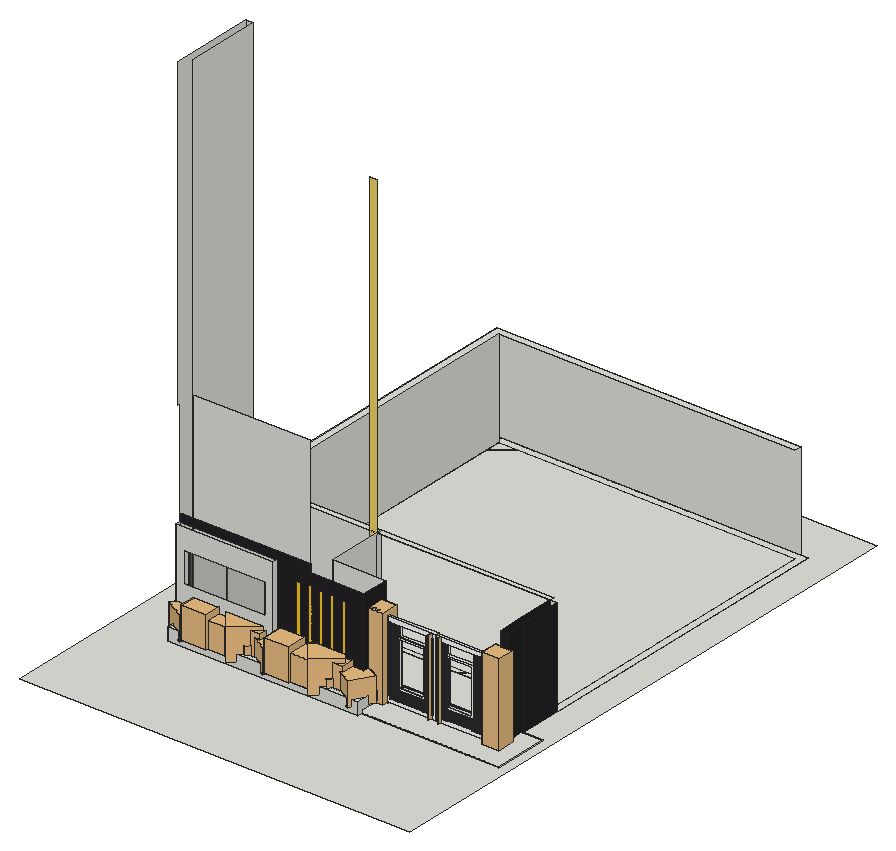
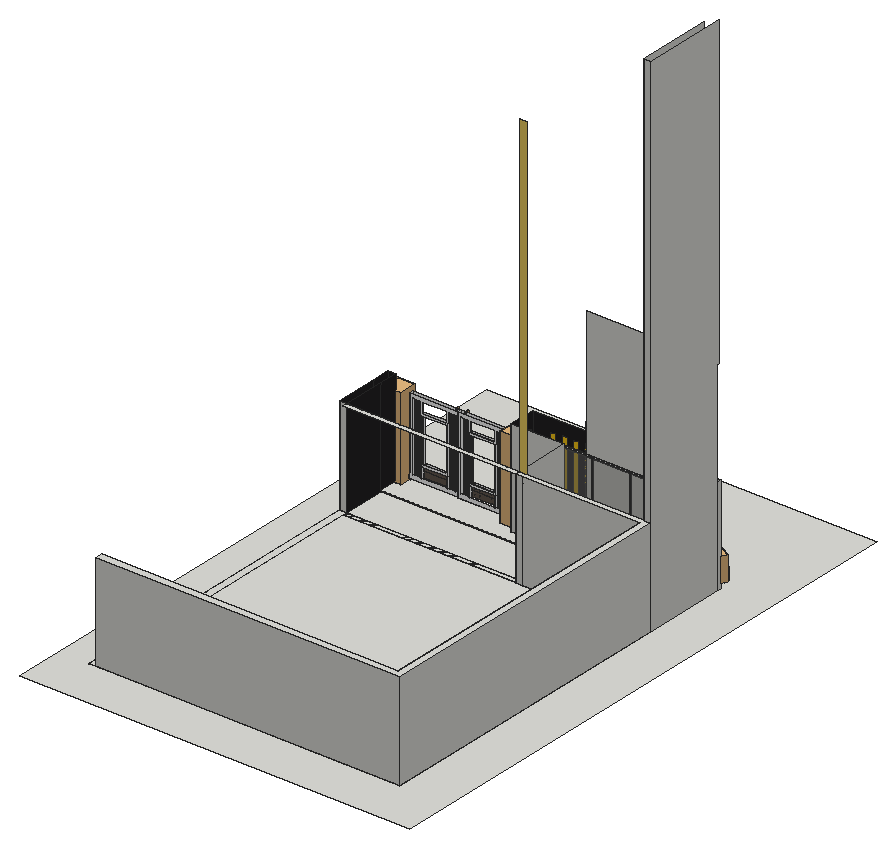
# SketchUp Ruby script. Lengths in inches.
U = 1.inch
M = Sketchup.active_model
def pt(a) = Geom::Point3d.new(a.map { |v| v * U })
def face(e, loops, mat)
  f = e.add_face(loops[0].map { |a| pt(a) })
  loops[1..].each { |l| e.add_face(l.map { |a| pt(a) }).erase! }
  f.material = f.back_material = mat if mat
  f
end
# faces: each face lists its corners as indices into pts; further lists are holes
def faces(e, pts, list, mat = nil) = list.each { |f| face(e, (f[0].is_a?(Array) ? f : [f]).map { |l| l.map { |i| pts[i] } }, mat) }
# xy, xz, yz: faces in a plane at the given z, y or x. An outline is a flat list of corners, or four numbers for a rectangle; further outlines are holes
def ring(l) = l.size == 4 ? [[l[0], l[1]], [l[2], l[1]], [l[2], l[3]], [l[0], l[3]]] : l.each_slice(2).to_a
def flat(e, list, mat, &to3) = list.each { |f| face(e, (f[0].is_a?(Array) ? f : [f]).map { |l| ring(l).map { |u, v| to3.(u, v) } }, mat) }
def xy(e, z, list, mat = nil) = flat(e, list, mat) { |x, y| [x, y, z] }
def xz(e, y, list, mat = nil) = flat(e, list, mat) { |x, z| [x, y, z] }
def yz(e, x, list, mat = nil) = flat(e, list, mat) { |y, z| [x, y, z] }
def lines(e, pts, list) = list.each { |a, b| e.add_line(pt(pts[a]), pt(pts[b])) }
# prism: a flat outline (further loops are holes) pulled along v
def prism(e, loops, v, mat = nil)
  f = face(e, loops, mat); d = Geom::Vector3d.new(v.map { |x| x * U })
  f.pushpull(f.normal.samedirection?(d) ? d.length : -d.length)
end
def box(e, o, s, mat = nil) = prism(e, [[o, [o[0] + s[0], o[1], o[2]], [o[0] + s[0], o[1] + s[1], o[2]], [o[0], o[1] + s[1], o[2]]]], [0, 0, s[2]], mat)
def at(x, y, z, deg = 0) = Geom::Transformation.translation(pt([x, y, z])) * Geom::Transformation.rotation(ORIGIN, Z_AXIS, deg.degrees)
def axes(o, x, y, z) = Geom::Transformation.new([*x, 0, *y, 0, *z, 0, *pt(o).to_a, 1])
def part(name) = M.definitions.add(name)
# library, detail: a bought-in or finely detailed component or shape, given as its bounding box
def library(name, o, s) = part(name).tap { |d| box(d.entities, o, s) }
def detail(e, o, s) = box(e.add_group.entities, o, s)
def put(e, d, t, mat = nil) = e.add_instance(d, t).tap { |i| i.material = mat if mat }
def group(e, t, mat = nil) = e.add_group.tap { |g| g.transformation = t; g.material = mat if mat }.entities
root = M.entities
M.materials.add("Glass_Mirror_3").color = [244, 212, 100]
M.materials.add("Marble_07_1K").color = [36, 34, 36]
M.materials.add("Material__1").color = [95, 70, 46]
M.materials.add("Metal_Perforated_08_1K").color = [255, 206, 27]
M.materials.add("[Color M00]").color = [255, 255, 255]
M.materials.add("[Color_000]").color = [255, 255, 255]
M.materials.add("[Color_C20]").color = [102, 91, 81]
M.materials.add("[Translucent Glass Gray]").color = [128, 128, 128]
M.materials["[Translucent Glass Gray]"].alpha = 0.29
c1 = library("Areca palm plant",[0,0,0],[49.1,36.6,54.46])
c2 = part("W1")
xy(c2.entities,15,[[0,0,2,198]])
xy(c2.entities,102.0625,[[0,0,2,198]],"[Color M00]")
xz(c2.entities,0,[[0,15,2,102.0625]],"[Color M00]")
xz(c2.entities,198,[[0,15,2,102.0625]])
yz(c2.entities,0,[[0.84,16,39.43,101.0625],[40.28,16,78.87,101.0625],[79.71,16,118.3,101.0625],[119.14,16,157.73,101.0625],[158.58,16,197.16,101.0625]])
yz(c2.entities,0,[[[0,15,198,102.0625],[0.84,16,197.16,101.0625]],[39.43,16,40.28,101.0625],[78.87,16,79.71,101.0625],[118.3,16,119.14,101.0625],[157.73,16,158.58,101.0625]],"[Color M00]")
yz(c2.entities,2,[[0.84,16,39.43,101.0625],[40.28,16,78.87,101.0625],[79.71,16,118.3,101.0625],[119.14,16,157.73,101.0625],[158.58,16,197.16,101.0625]])
yz(c2.entities,2,[[[0,15,198,102.0625],[0.84,16,197.16,101.0625]],[39.43,16,40.28,101.0625],[78.87,16,79.71,101.0625],[118.3,16,119.14,101.0625],[157.73,16,158.58,101.0625]],"[Color M00]")
c3 = library("Group\#74",[-84.69,-90.07,-0.36],[176.51,175.13,171.4])
c4 = library("Group20\#1",[-20.81,-17.08,3.79],[39.86,39.43,37.51])
c5 = library("Group\#130",[-7.34,-1.2,0],[38.67,35.81,49.04])
c6 = library("Group38\#2",[14.01,28.44,-23.43],[18.58,18.32,38.89])
c7 = part("PLANTS (1)")
put(c7.entities,c1,axes([38.49,169.84,6.02],[0.45017,-0.56191,0],[0.66137,0.52986,0],[0,0,0.72]))
put(c7.entities,c1,axes([38.49,68.02,6.02],[0.45017,-0.56191,0],[0.66137,0.52986,0],[0,0,0.72]))
put(c7.entities,c2,axes([76.68,11.43,-0.0625],[1,0,0],[0,1.18586,0],[0,0,1]),"[Translucent Glass Gray]")
put(c7.entities,c3,axes([59.61,184.54,5.99],[-0.04961,-0.08593,0],[0.08593,-0.04961,0],[0,0,0.10522]))
put(c7.entities,c3,axes([59.61,204.61,5.99],[-0.04961,-0.08593,0],[0.08593,-0.04961,0],[0,0,0.10522]))
put(c7.entities,c3,axes([59.61,157.29,5.99],[-0.04961,-0.08593,0],[0.08593,-0.04961,0],[0,0,0.10522]))
put(c7.entities,c4,axes([63.65,91.4,4.71],[0,0.85,0],[-0.85,0,0],[0,0,0.85]))
put(c7.entities,c5,axes([69.62,101.34,7.93],[0,0.79,0],[-0.79,0,0],[0,0,0.79]))
put(c7.entities,c6,axes([40.58,10.27,28.11],[0.8848,0,0],[0,0.94674,0],[0,0,0.85826]))
put(c7.entities,c3,axes([59.61,55.48,5.99],[-0.04961,-0.08593,0],[0.08593,-0.04961,0],[0,0,0.10522]))
put(c7.entities,c3,axes([59.61,82.73,5.99],[-0.04961,-0.08593,0],[0.08593,-0.04961,0],[0,0,0.10522]))
put(c7.entities,c3,axes([61.875,132.66,6.01],[-0.08133,-0.14087,0],[0.14087,-0.08133,0],[0,0,0.1725]))
put(c7.entities,c3,axes([59.61,102.79,5.99],[-0.04961,-0.08593,0],[0.08593,-0.04961,0],[0,0,0.10522]))
put(c7.entities,c3,axes([61.875,27.22,6.01],[-0.08133,-0.14087,0],[0.14087,-0.08133,0],[0,0,0.1725]))
put(c7.entities,c3,axes([61.875,234.47,6.01],[-0.08133,-0.14087,0],[0.14087,-0.08133,0],[0,0,0.1725]))
put(c7.entities,c5,axes([69.62,203.15,7.93],[0,0.79,0],[-0.79,0,0],[0,0,0.79]))
put(c7.entities,c4,axes([63.65,193.21,4.71],[0,0.85,0],[-0.85,0,0],[0,0,0.85]))
put(c7.entities,c6,axes([40.58,112.08,28.11],[0.8848,0,0],[0,0.94674,0],[0,0,0.85826]))
g1 = group(c7.entities,at(44.68,11.43,-0.0625))
xy(g1,0,[[0,0,6,234.8],[30,0,36,234.8]])
xy(g1,3,[[6,0,30,234.8]])
xy(g1,7,[[6,5,30,229.8]],"Material__1")
xy(g1,15,[[[0,0,36,234.8],[6,5,30,229.8]]])
xz(g1,0,[[0,0,6,0,6,3,30,3,30,0,36,0,36,15,0,15]])
xz(g1,5,[[6,7,30,15]])
xz(g1,229.8,[[6,7,30,15]])
xz(g1,234.8,[[0,0,0,15,36,15,36,0,30,0,30,3,6,3,6,0]])
yz(g1,0,[[0,0,234.8,15]])
yz(g1,6,[[0,0,234.8,3],[5,7,229.8,15]])
yz(g1,30,[[0,0,234.8,3],[5,7,229.8,15]])
yz(g1,36,[[0,0,234.8,15]])
c8 = library("Gate pillar",[0,0,0],[97.06,71.13,326.45])
c9 = library("Gate pull handle",[-0.01,0,0],[1.26,2.875,48])
c10 = part("Gate slat")
xy(c10.entities,0,[[0.39,114.16,6.3,114.17]])
xy(c10.entities,0,[[0.39,0,6.3,114.16]],"[Color_C20]")
xy(c10.entities,0.39,[[0.39,0,0.79,114.17],[0.98,0,2.07,114.17],[2.36,0,3.2,114.17],[3.59,0,4.37,114.17],[4.56,0,5.71,114.17],
  [5.91,0,6.3,114.17]],"[Color_C20]")
xy(c10.entities,0.79,[[0.39,0,0.79,114.17],[0.98,0,2.07,114.17],[2.36,0,3.2,114.17],[3.59,0,4.37,114.17],[4.56,0,5.71,114.17],
  [5.91,0,6.3,114.17]],"[Color_C20]")
xy(c10.entities,0.99,[[1.13,0,1.21,114.16],[1.87,0,1.94,114.16],[2.61,0,2.68,114.16],[3.35,0,3.42,114.16],[4.08,0,4.16,114.16],
  [4.82,0,4.9,114.16],[5.5625,0,5.63,114.16],[6.3,0,6.37,114.16]],"[Color_C20]")
xy(c10.entities,1.18,[[0.39,114.16,3.35,114.17],[3.35,114.16,6.3,114.17]])
xy(c10.entities,1.18,[[0.39,0,1.13,114.16],[1.21,0,1.87,114.16],[1.94,0,2.61,114.16],[2.68,0,3.35,114.16],[3.42,0,4.08,114.16],
  [4.16,0,4.82,114.16],[4.9,0,5.5625,114.16],[5.63,0,6.3,114.16]],"[Color_C20]")
xz(c10.entities,0,[[[0.39,0,6.3,0,6.3,0.39,5.91,0.39,5.91,0.79,6.3,0.79,6.3,1.18,5.63,1.18,5.63,0.99,5.5625,0.99,5.5625,1.18,4.9,1.18,4.9,0.99,4.82,0.99,4.82,1.18,4.16,1.18,4.16,0.99,4.08,0.99,4.08,1.18,3.42,1.18,3.42,0.99,3.35,0.99,3.35,1.18,2.68,1.18,2.68,0.99,2.61,0.99,2.61,1.18,1.94,1.18,1.94,0.99,1.87,0.99,1.87,1.18,1.21,1.18,1.21,0.99,1.13,0.99,1.13,1.18,0.39,1.18,0.39,0.79,0.79,0.79,0.79,0.39,0.39,0.39],[4.56,0.39,5.71,0.79],[0.98,0.39,2.07,0.79],[2.36,0.39,3.2,0.79],[3.59,0.39,4.37,0.79]],[6.3,0.99,6.37,1.18]],"[Color_C20]")
xz(c10.entities,114.16,[[1.13,0.99,1.21,1.18],[1.87,0.99,1.94,1.18],[2.61,0.99,2.68,1.18],[3.35,0.99,3.42,1.18],[4.08,0.99,4.16,1.18],
  [4.82,0.99,4.9,1.18],[5.5625,0.99,5.63,1.18]],"[Color_C20]")
xz(c10.entities,114.17,[[[0.39,0,0.39,0.39,0.79,0.39,0.79,0.79,0.39,0.79,0.39,1.18,6.3,1.18,6.3,0.79,5.91,0.79,5.91,0.39,6.3,0.39,6.3,0],[4.56,0.39,5.71,0.79],[0.98,0.39,2.07,0.79],[2.36,0.39,3.2,0.79],[3.59,0.39,4.37,0.79]]],"[Color_C20]")
yz(c10.entities,0.39,[[114.16,0,114.17,0.39],[114.16,0.79,114.17,1.18]])
yz(c10.entities,0.39,[[0,0,114.16,0.39],[0,0.79,114.16,1.18]],"[Color_C20]")
yz(c10.entities,0.79,[[0,0.39,114.17,0.79]],"[Color_C20]")
yz(c10.entities,0.98,[[0,0.39,114.17,0.79]],"[Color_C20]")
yz(c10.entities,1.13,[[0,0.99,114.16,1.18]],"[Color_C20]")
yz(c10.entities,1.21,[[0,0.99,114.16,1.18]],"[Color_C20]")
yz(c10.entities,1.87,[[0,0.99,114.16,1.18]],"[Color_C20]")
yz(c10.entities,1.94,[[0,0.99,114.16,1.18]],"[Color_C20]")
yz(c10.entities,2.07,[[0,0.39,114.17,0.79]],"[Color_C20]")
yz(c10.entities,2.36,[[0,0.39,114.17,0.79]],"[Color_C20]")
yz(c10.entities,2.61,[[0,0.99,114.16,1.18]],"[Color_C20]")
yz(c10.entities,2.68,[[0,0.99,114.16,1.18]],"[Color_C20]")
yz(c10.entities,3.2,[[0,0.39,114.17,0.79]],"[Color_C20]")
yz(c10.entities,3.35,[[0,0.99,114.16,1.18]],"[Color_C20]")
yz(c10.entities,3.42,[[0,0.99,114.16,1.18]],"[Color_C20]")
yz(c10.entities,3.59,[[0,0.39,114.17,0.79]],"[Color_C20]")
yz(c10.entities,4.08,[[0,0.99,114.16,1.18]],"[Color_C20]")
yz(c10.entities,4.16,[[0,0.99,114.16,1.18]],"[Color_C20]")
yz(c10.entities,4.37,[[0,0.39,114.17,0.79]],"[Color_C20]")
yz(c10.entities,4.56,[[0,0.39,114.17,0.79]],"[Color_C20]")
yz(c10.entities,4.82,[[0,0.99,114.16,1.18]],"[Color_C20]")
yz(c10.entities,4.9,[[0,0.99,114.16,1.18]],"[Color_C20]")
yz(c10.entities,5.5625,[[0,0.99,114.16,1.18]],"[Color_C20]")
yz(c10.entities,5.63,[[0,0.99,114.16,1.18]],"[Color_C20]")
yz(c10.entities,5.71,[[0,0.39,114.17,0.79]],"[Color_C20]")
yz(c10.entities,5.91,[[0,0.39,114.17,0.79]],"[Color_C20]")
yz(c10.entities,6.3,[[114.16,0,114.17,0.39],[114.16,0.79,114.17,1.18]])
yz(c10.entities,6.3,[[0,0,114.16,0.39],[0,0.79,114.16,0.99],[0,0.99,114.16,1.18]],"[Color_C20]")
yz(c10.entities,6.37,[[0,0.99,114.16,1.18]],"[Color_C20]")
p = [[0,0,0],[0.39,0,0]]
lines(c10.entities,p,[[0,1]])
c11 = part("Vertical gate panel")
put(c11.entities,c10,axes([0,1.18,0],[3.67755,0,0],[0,0,2.40086],[0,-1,0]))
put(c11.entities,c10,axes([21.72,1.18,0],[3.67755,0,0],[0,0,2.40086],[0,-1,0]))
box(root,[270.54,152.64,0],[198.16,66.55,0.89])
xy(root,0,[[[0,0,480,720],[60.23,165,60.23,171,60,171,60,660,444,660,444,220.51,435,220.22,435,180,287.05,180,287.05,171,180,171,180,165]],[60.23,165,180,165,180,171,287.05,171,287.05,180,69,180,69,273,60,273,60,171,60.23,171],[69,180,213,273],[213,180,222,272.89],[222,180,287.05,204.3],
  [287.05,180,435,180,435,273,222,273,222,204.3,287.05,204.3],[213,272.89,222,273],[60,273,444,660]])
xy(root,0.89,[[426.7,183.89,426.59,183.91,426.48,183.96,426.39,184.05,426.33,184.16,426.28,184.29,426.27,184.43,426.28,184.57,426.33,184.7,426.39,184.8125,426.48,184.9,426.59,184.95,426.7,184.97,426.81,184.95,426.91,184.9,427,184.8125,427.07,184.7,427.11,184.57,427.13,184.43,427.11,184.29,427.07,184.16,427,184.05,426.91,183.96,426.81,183.91],[306.7,184.02,306.59,184.04,306.49,184.09,306.4,184.1875,306.33,184.31,306.29,184.45,306.27,184.6,306.29,184.75,306.33,184.89,306.4,185.01,306.49,185.1,306.59,185.16,306.7,185.18,306.8125,185.16,306.92,185.1,307.01,185.01,307.08,184.89,307.12,184.75,307.13,184.6,307.12,184.45,307.08,184.31,307.01,184.1875,306.92,184.09,306.8125,184.04]])
xy(root,2.74,[[[304.88,182.1,366.58,186.51],[306.7,184.02,306.8125,184.04,306.92,184.09,307.01,184.1875,307.08,184.31,307.12,184.45,307.13,184.6,307.12,184.75,307.08,184.89,307.01,185.01,306.92,185.1,306.8125,185.16,306.7,185.18,306.59,185.16,306.49,185.1,306.4,185.01,306.33,184.89,306.29,184.75,306.27,184.6,306.29,184.45,306.33,184.31,306.4,184.1875,306.49,184.09,306.59,184.04]],[[366.83,182.1,427.35,186.22],[426.7,183.89,426.81,183.91,426.91,183.96,427,184.05,427.07,184.16,427.11,184.29,427.13,184.43,427.11,184.57,427.07,184.7,427,184.8125,426.91,184.9,426.81,184.95,426.7,184.97,426.59,184.95,426.48,184.9,426.39,184.8125,426.33,184.7,426.28,184.57,426.27,184.43,426.28,184.29,426.33,184.16,426.39,184.05,426.48,183.96,426.59,183.91]]],"[Color_000]")
xy(root,7.51,[[320.1875,182.1,321.64,182.83],[321.64,182.1,352.12,182.83],[352.12,182.1,353.58,182.83],[379.83,182.1,381.28,182.78],[381.28,182.1,411.76,182.78],
  [411.76,182.1,413.21,182.78]])
xy(root,7.51,[[310.6,182.1,315.39,186.51],[315.39,182.1,320.1875,186.51],[353.58,182.1,363.16,182.83],[370.24,182.1,379.83,182.78],[413.21,182.1,418.01,186.22],
  [418.01,182.1,422.8,186.22],[370.24,182.78,379.83,186.22],[381.28,182.78,411.76,186.22],[321.64,182.83,352.12,186.51],[353.58,182.83,363.16,186.51]],"[Color_000]")
xy(root,9.32,[[304.88,182.1,307.1875,186.51],[426.21,182.1,427.35,186.22]],"[Color_000]")
xy(root,20.93,[[321.64,182.1,352.12,186.51],[381.28,182.1,411.76,186.22]],"[Color_000]")
xz(root,165,[[[60.23,0,180,120],[69.92,57.77,170.46,95.29]]])
xz(root,171,[[[60,0,60.23,0,60.23,120,180,120,180,0,287.05,0,287.05,120,222,120,222,130,60,130],[203.49,11.18,208.91,105.4],[217.4,12.02,222.82,106.24],[230.94,10.375,236.37,104.6],[244.77,10.53,250.19,104.75],[259.62,9.05,265.04,103.27]]],"Marble_07_1K")
xz(root,171,[[259.62,9.05,265.04,103.27],[230.94,10.375,236.37,104.6],[244.77,10.53,250.19,104.75],[203.49,11.18,208.91,105.4],[217.4,12.02,222.82,106.24]],"Metal_Perforated_08_1K")
xz(root,180,[[69,0,213,259.85]])
xz(root,182.1,[[[304.88,2.74,366.58,2.74,366.58,97.49,307.1875,97.49,307.1875,9.32,304.88,9.32],[310.6,7.51,363.16,92.71]],[[366.83,2.74,427.35,2.74,427.35,9.32,426.21,9.32,426.21,97.49,366.83,97.49],[370.24,7.51,422.8,92.71]],[320.1875,7.51,321.64,20.93],[352.12,7.51,353.58,20.93],[379.83,7.51,381.28,20.93],
  [411.76,7.51,413.21,20.93],[320.1875,20.93,353.58,20.93,353.58,79.29,320.1875,79.29,320.1875,77.25,352.12,77.25,352.12,22.97,321.64,22.97,321.64,77.25,320.1875,77.25],[379.83,20.93,413.21,20.93,413.21,77.25,411.76,77.25,411.76,22.97,381.28,22.97,381.28,77.25,413.21,77.25,413.21,79.29,379.83,79.29]],"[Color_000]")
xz(root,186.22,[[[366.83,2.74,366.83,97.49,426.21,97.49,426.21,9.32,427.35,9.32,427.35,2.74],[381.28,22.97,411.76,77.25],[413.21,7.51,422.8,92.71],[370.24,7.51,379.83,92.71],[381.28,79.29,411.76,92.71],[381.28,7.51,411.76,20.93]]],"[Color_000]")
xz(root,186.51,[[[304.88,2.74,304.88,9.32,307.1875,9.32,307.1875,97.49,366.58,97.49,366.58,2.74],[321.64,22.97,352.12,77.25],[310.6,7.51,320.1875,92.71],[353.58,7.51,363.16,92.71],[321.64,79.29,352.12,92.71],[321.64,7.51,352.12,20.93]]],"[Color_000]")
xz(root,204.3,[[222,0,287.05,120]])
xz(root,272.89,[[213,0,222,509.54]],"Glass_Mirror_3")
xz(root,273,[[60,0,69,629.54],[435,0,444,120]])
yz(root,60,[[171,0,171,249.85,168,249.85,168,629.54,273,629.54,273,0]])
yz(root,60.23,[[165,0,171,120]])
yz(root,69,[[180,0,273,629.54]])
yz(root,180,[[165,0,171,120]])
yz(root,222,[[204.3,0,272.89,120]])
yz(root,287.05,[[171,0,204.3,120]],"Marble_07_1K")
yz(root,304.88,[[182.1,2.74,186.51,9.32]],"[Color_000]")
yz(root,307.1875,[[[182.1,9.32,186.51,97.49],[183.66,79.68,185.32,82.91],[183.66,84.2,185.32,87.3125],[183.66,83.06,185.32,84.04]]],"[Color_000]")
yz(root,310.6,[[182.1,7.51,186.51,92.71]],"[Color_000]")
yz(root,320.1875,[[182.1,7.51,186.51,20.93],[182.1,20.93,186.51,77.25]],"[Color_000]")
yz(root,321.64,[[182.1,7.51,186.51,20.93]],"[Color_000]")
yz(root,352.12,[[182.1,7.51,186.51,20.93]],"[Color_000]")
yz(root,353.58,[[182.1,7.51,186.51,20.93],[182.1,20.93,186.51,79.29]],"[Color_000]")
yz(root,363.16,[[182.1,7.51,186.51,92.71]],"[Color_000]")
yz(root,366.58,[[182.1,2.74,186.51,97.49]],"[Color_000]")
yz(root,366.83,[[182.1,2.74,186.22,97.49]],"[Color_000]")
yz(root,370.24,[[182.1,7.51,186.22,92.71]],"[Color_000]")
yz(root,379.83,[[182.1,7.51,186.22,20.93],[182.1,20.93,186.22,79.29]],"[Color_000]")
yz(root,381.28,[[182.1,7.51,186.22,20.93]],"[Color_000]")
yz(root,411.76,[[182.1,7.51,186.22,20.93]],"[Color_000]")
yz(root,413.21,[[182.1,7.51,186.22,20.93],[182.1,20.93,186.22,77.25]],"[Color_000]")
yz(root,422.8,[[182.1,7.51,186.22,92.71]],"[Color_000]")
yz(root,426.21,[[[182.1,9.32,186.22,97.49],[183.55,79.68,183.55,82.91,185.11,82.91,185.11,83.06,183.55,83.06,183.55,84.04,185.11,84.04,185.11,79.68],[183.55,84.2,185.11,87.3125]]],"[Color_000]")
yz(root,427.35,[[182.1,2.74,186.22,9.32]],"[Color_000]")
yz(root,435,[[220.22,0,273,120]],"Marble_07_1K")
yz(root,444,[[220.51,0,273,120]],"Marble_07_1K")
p = [[444,220.51,0],[444,220.51,1.41],[435,220.22,1.52],[435,220.22,0],[426.59,183.91,2.74],[426.48,183.96,2.74],
  [426.48,183.96,0.89],[426.59,183.91,0.89],[426.7,183.89,2.74],[426.7,183.89,0.89],[426.81,183.91,2.74],[426.81,183.91,0.89],
  [426.91,183.96,2.74],[426.91,183.96,0.89],[306.59,184.04,2.74],[306.49,184.09,2.74],[306.49,184.09,0.89],[306.59,184.04,0.89],
  [306.7,184.02,2.74],[306.7,184.02,0.89],[306.8125,184.04,2.74],[306.8125,184.04,0.89],[306.92,184.09,2.74],[306.92,184.09,0.89],
  [426.39,184.05,2.74],[426.33,184.16,2.74],[426.33,184.16,0.89],[426.39,184.05,0.89],[427,184.05,2.74],[427,184.05,0.89],
  [427.07,184.16,2.74],[427.07,184.16,0.89],[306.4,184.1875,2.74],[306.4,184.1875,0.89],[307.01,184.1875,2.74],[307.01,184.1875,0.89],
  [306.33,184.31,2.74],[306.33,184.31,0.89],[307.08,184.31,2.74],[307.08,184.31,0.89],[426.28,184.29,2.74],[426.28,184.29,0.89],
  [427.11,184.29,2.74],[427.11,184.29,0.89],[306.29,184.45,2.74],[306.29,184.45,0.89],[307.12,184.45,2.74],[307.12,184.45,0.89],
  [426.27,184.43,2.74],[426.27,184.43,0.89],[427.13,184.43,2.74],[427.13,184.43,0.89],[306.27,184.6,2.74],[306.27,184.6,0.89],
  [307.13,184.6,2.74],[307.13,184.6,0.89],[426.28,184.57,2.74],[426.28,184.57,0.89],[427.11,184.57,2.74],[427.11,184.57,0.89],
  [306.29,184.75,2.74],[306.29,184.75,0.89],[307.12,184.75,2.74],[307.12,184.75,0.89],[426.33,184.7,2.74],[426.33,184.7,0.89],
  [427.07,184.7,2.74],[427.07,184.7,0.89],[306.33,184.89,2.74],[306.33,184.89,0.89],[307.08,184.89,2.74],[307.08,184.89,0.89],
  [426.39,184.8125,2.74],[426.39,184.8125,0.89],[427,184.8125,2.74],[427,184.8125,0.89],[426.48,184.9,2.74],[426.48,184.9,0.89],
  [426.91,184.9,2.74],[426.91,184.9,0.89],[306.4,185.01,2.74],[306.4,185.01,0.89],[307.01,185.01,2.74],[307.01,185.01,0.89],
  [426.59,184.95,2.74],[426.59,184.95,0.89],[426.81,184.95,2.74],[426.81,184.95,0.89],[306.49,185.1,2.74],[306.49,185.1,0.89],
  [306.92,185.1,2.74],[306.92,185.1,0.89],[426.7,184.97,2.74],[426.7,184.97,0.89],[306.59,185.16,2.74],[306.59,185.16,0.89],
  [306.8125,185.16,2.74],[306.8125,185.16,0.89],[306.7,185.18,2.74],[306.7,185.18,0.89],[444.75,197.01,1.41],[435.75,196.73,1.52],
  [435.75,196.73,120],[444.75,197.01,120],[444,220.51,120],[435,220.22,120],[442.11,171,0],[444,171,0],
  [287.05,171,0],[398.96,171,0],[437.08,219.19,0.89],[446.08,219.19,0.89],[401.04,180,0],[413.82,182.78,7.51],
  [413.21,182.78,7.51],[319.58,182.83,7.51],[320.1875,182.83,7.51],[366.58,182.1,2.74],[366.83,182.1,2.74]]
faces(root,p,[[0,1,2,3],[2,1,100,101]])
faces(root,p,[[4,5,6,7],[8,4,7,9],[10,8,9,11],[12,10,11,13],[14,15,16,17],[18,14,17,19],[20,18,19,21],[22,20,21,23],
  [24,25,26,27],[5,24,27,6],[28,12,13,29],[30,28,29,31],[15,32,33,16],[34,22,23,35],[32,36,37,33],[38,34,35,39],
  [25,40,41,26],[42,30,31,43],[36,44,45,37],[46,38,39,47],[40,48,49,41],[50,42,43,51],[44,52,53,45],[54,46,47,55],
  [48,56,57,49],[58,50,51,59],[52,60,61,53],[62,54,55,63],[56,64,65,57],[66,58,59,67],[60,68,69,61],[70,62,63,71],
  [64,72,73,65],[74,66,67,75],[72,76,77,73],[78,74,75,79],[68,80,81,69],[82,70,71,83],[76,84,85,77],[86,78,79,87],
  [80,88,89,81],[90,82,83,91],[84,92,93,85],[92,86,87,93],[88,94,95,89],[96,90,91,97],[94,98,99,95],[98,96,97,99]],"[Color_000]")
faces(root,p,[[102,101,100,103],[1,104,103,100],[105,2,101,102]],"Marble_07_1K")
lines(root,p,[[106,107],[108,109],[110,111],[109,106],[109,112],[113,114],[115,116],[117,118]])
g2 = group(root,at(60,273,0))
p = [[153,6,0],[375,6,0],[375,378,0],[153,0,0],[9,0,0],[384,387,0],
  [384,0,0],[0,0,0],[0,387,0],[9,378,0],[375,0,0],[9,6,0],
  [162,0,0]]
lines(g2,p,[[0,1],[1,2],[3,4],[5,6],[4,7],[8,5],[2,9],[7,8],[6,10],[9,11],[11,0],[10,12]])
g3 = group(root,at(60,273,0))
xy(g3,0,[[0,0,162,0,162,6,9,6,9,378,375,378,375,387,0,387],[375,0,384,0,384,387,375,387,375,378,9,378,9,6,375,6],[162,0,375,6]])
xy(g3,120,[[162,-0.11,375,0],[0,0,162,0,162,6,9,6,9,378,375,378,375,387,0,387],[162,0,375,6]])
xz(g3,0,[[0,0,9,120]])
xz(g3,6,[[9,0,153,120],[153,0,162,120]])
xz(g3,387,[[0,0,375,120]])
yz(g3,0,[[0,0,387,120]])
yz(g3,9,[[6,0,378,120]])
yz(g3,162,[[-0.11,0,6,120]])
put(root,c7,at(310.14,102.86,0.0625,90))
put(root,c8,axes([284.32,176.85,0.89],[0.22204,0,0],[0,0.299,0],[0,0,0.31083]))
put(root,c8,axes([449.08,176.85,0.89],[-0.22204,0,0],[0,0.299,0],[0,0,0.31083]))
put(root,c9,axes([373.18,178.51,3.12],[-0.95479,0,0],[0,1.24954,0],[0,0,1.96607]))
put(root,c9,axes([360.22,178.25,3.12],[0.95479,0,0],[0,1.339,0],[0,0,1.96607]))
put(root,c11,axes([381.28,182.78,7.05],[0,0,0.31699],[0,0.27902,0],[0.11119,0,0]))
put(root,c11,axes([352.12,182.83,7.05],[0,0,0.31699],[0,0.299,0],[-0.11119,0,0]))
put(root,c10,axes([423.18,183.11,7.51],[-0.81658,0,0],[0,0,0.74625],[0,-0.27902,0]))
put(root,c10,axes([418.36,183.11,7.51],[-0.81658,0,0],[0,0,0.74625],[0,-0.27902,0]))
put(root,c10,axes([375.38,183.11,7.51],[-0.81658,0,0],[0,0,0.74625],[0,-0.27902,0]))
put(root,c10,axes([380.2,183.11,7.51],[-0.81658,0,0],[0,0,0.74625],[0,-0.27902,0]))
put(root,c10,axes([310.22,183.19,7.51],[0.81658,0,0],[0,0,0.74625],[0,-0.299,0]))
put(root,c10,axes([315.04,183.19,7.51],[0.81658,0,0],[0,0,0.74625],[0,-0.299,0]))
put(root,c10,axes([353.2,183.19,7.51],[0.81658,0,0],[0,0,0.74625],[0,-0.299,0]))
put(root,c10,axes([358.02,183.19,7.51],[0.81658,0,0],[0,0,0.74625],[0,-0.299,0]))
